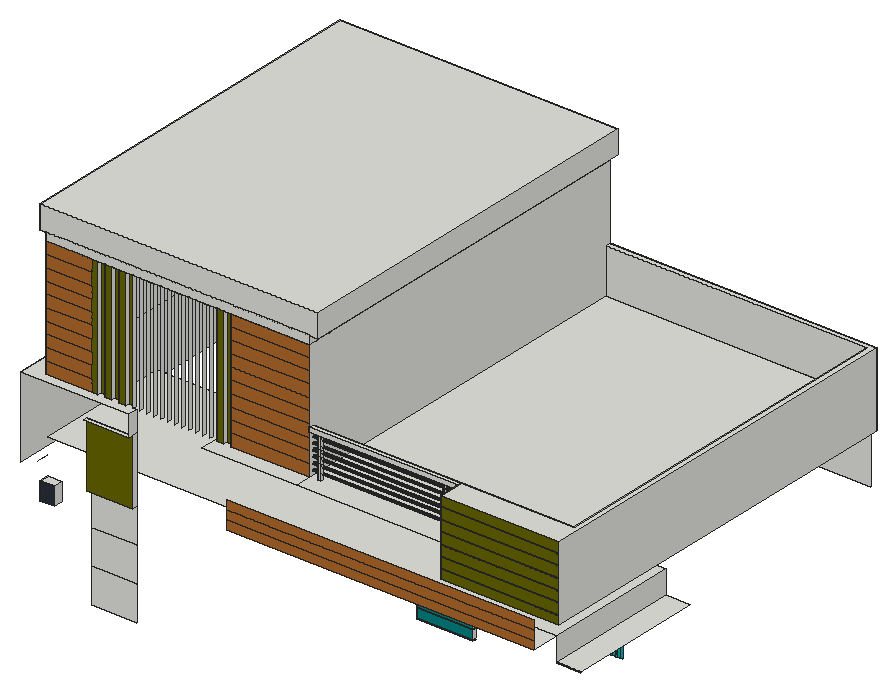
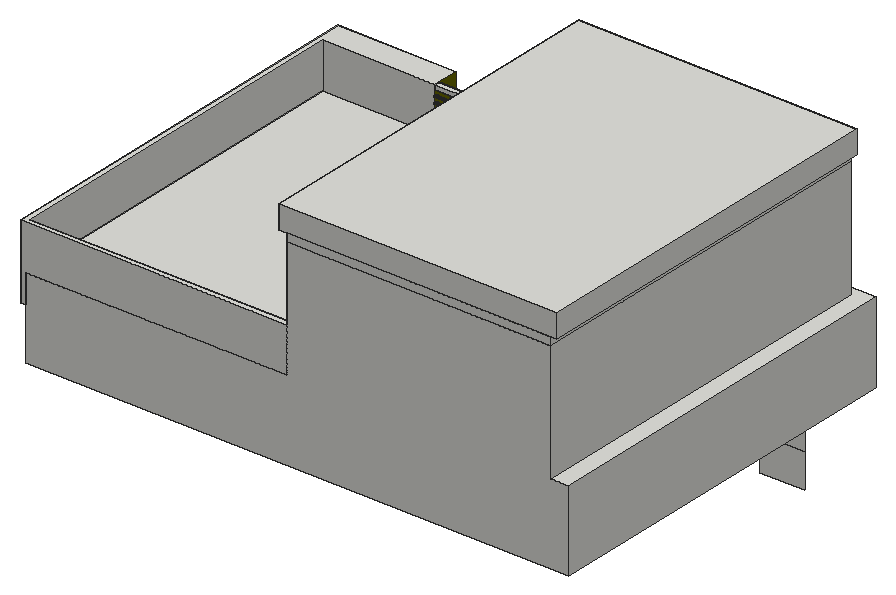
# SketchUp Ruby script. Lengths in inches.
U = 1.inch
M = Sketchup.active_model
def pt(a) = Geom::Point3d.new(a.map { |v| v * U })
def face(e, loops, mat)
  f = e.add_face(loops[0].map { |a| pt(a) })
  loops[1..].each { |l| e.add_face(l.map { |a| pt(a) }).erase! }
  f.material = f.back_material = mat if mat
  f
end
# faces: each face lists its corners as indices into pts; further lists are holes
def faces(e, pts, list, mat = nil) = list.each { |f| face(e, (f[0].is_a?(Array) ? f : [f]).map { |l| l.map { |i| pts[i] } }, mat) }
# xy, xz, yz: faces in a plane at the given z, y or x. An outline is a flat list of corners, or four numbers for a rectangle; further outlines are holes
def ring(l) = l.size == 4 ? [[l[0], l[1]], [l[2], l[1]], [l[2], l[3]], [l[0], l[3]]] : l.each_slice(2).to_a
def flat(e, list, mat, &to3) = list.each { |f| face(e, (f[0].is_a?(Array) ? f : [f]).map { |l| ring(l).map { |u, v| to3.(u, v) } }, mat) }
def xy(e, z, list, mat = nil) = flat(e, list, mat) { |x, y| [x, y, z] }
def xz(e, y, list, mat = nil) = flat(e, list, mat) { |x, z| [x, y, z] }
def yz(e, x, list, mat = nil) = flat(e, list, mat) { |y, z| [x, y, z] }
def lines(e, pts, list) = list.each { |a, b| e.add_line(pt(pts[a]), pt(pts[b])) }
# prism: a flat outline (further loops are holes) pulled along v
def prism(e, loops, v, mat = nil)
  f = face(e, loops, mat); d = Geom::Vector3d.new(v.map { |x| x * U })
  f.pushpull(f.normal.samedirection?(d) ? d.length : -d.length)
end
def box(e, o, s, mat = nil) = prism(e, [[o, [o[0] + s[0], o[1], o[2]], [o[0] + s[0], o[1] + s[1], o[2]], [o[0], o[1] + s[1], o[2]]]], [0, 0, s[2]], mat)
def at(x, y, z, deg = 0) = Geom::Transformation.translation(pt([x, y, z])) * Geom::Transformation.rotation(ORIGIN, Z_AXIS, deg.degrees)
def axes(o, x, y, z) = Geom::Transformation.new([*x, 0, *y, 0, *z, 0, *pt(o).to_a, 1])
def part(name) = M.definitions.add(name)
# library, detail: a bought-in or finely detailed component or shape, given as its bounding box
def library(name, o, s) = part(name).tap { |d| box(d.entities, o, s) }
def detail(e, o, s) = box(e.add_group.entities, o, s)
def put(e, d, t, mat = nil) = e.add_instance(d, t).tap { |i| i.material = mat if mat }
def group(e, t, mat = nil) = e.add_group.tap { |g| g.transformation = t; g.material = mat if mat }.entities
root = M.entities
M.materials.add("[Color E08]").color = [102, 102, 0]
M.materials.add("[Color H06]").color = [0, 170, 170]
M.materials.add("[Color H07]").color = [0, 132, 132]
M.materials.add("[Tile Navy]").color = [43, 47, 58]
M.materials.add("[Wood Bamboo]").color = [177, 105, 43]
xy(root,176.551,[[244.901,188.3125,281.433,190.25]])
xy(root,177.301,[[244.901,188.3125,281.433,190.25]])
xy(root,182.734,[[244.901,188.3125,281.433,190.25]])
xy(root,183.484,[[244.901,188.3125,281.433,190.25]])
xy(root,188.918,[[244.901,188.3125,281.433,190.25]])
xy(root,189.668,[[244.901,188.3125,281.433,190.25]])
xy(root,195.101,[[244.901,188.3125,281.433,190.25]])
xy(root,195.851,[[219.446,181.4375,232.76,188.3125],[244.901,188.3125,281.433,190.25]])
xy(root,201.284,[[244.901,188.3125,281.433,190.25]])
xy(root,202.034,[[244.901,188.3125,281.433,190.25]])
xy(root,207.467,[[244.901,188.3125,281.433,190.25]])
xy(root,207.989,[[308.71,183.8125,317.574,188.3125]])
xy(root,208.217,[[244.901,188.3125,281.433,190.25]])
xy(root,208.654,[[368.197,183.8125,377.586,188.3125]])
xy(root,209.164,[[219.446,181.4375,232.76,188.3125]])
xy(root,213.65,[[244.901,188.3125,281.433,190.25]])
xy(root,214.4,[[244.901,188.3125,281.433,190.25]])
xy(root,218.86,[[308.447,183.8125,323.522,188.3125],[323.522,183.8125,361.655,188.3125],[361.655,183.8125,378.322,188.3125]])
xy(root,219.833,[[244.901,188.3125,281.433,190.25]])
xy(root,220.583,[[244.901,188.3125,281.433,190.25]])
xy(root,226.016,[[244.901,188.3125,281.433,190.25]])
xy(root,226.766,[[244.901,188.3125,281.433,190.25]])
xy(root,232.199,[[244.901,188.3125,281.433,190.25]])
xy(root,232.949,[[244.901,188.3125,281.433,190.25]])
xy(root,234.298,[[308.447,183.8125,378.322,188.3125]])
xy(root,237.467,[[244.901,188.3125,281.433,190.25]])
xy(root,237.5,[[89.426,80,98.551,86.125]])
xy(root,238.982,[[243.386,188.3125,282.948,190.25]])
xy(root,239.5,[[302.454,183.8125,382.891,188.3125]])
xy(root,246.5625,[[405.1875,100.496,421.0625,188.3125]])
xy(root,247.247,[[112.439,89,141.564,92.3125]])
xy(root,249,[[89.426,80,98.551,86.125]])
xy(root,261.3125,[[207.779,82.0625,405.1875,100.496],[77.779,100.496,405.1875,188.3125]])
xy(root,284.3125,[[348.593,77.9375,348.593,82.0625,421.0625,82.0625,421.0625,333.5625,424.6875,333.5625,424.6875,77.9375]])
xy(root,289.375,[[112.439,86.125,141.564,89]])
xy(root,290,[[348.593,77.9375,424.6875,78.25]])
xy(root,290.5625,[[348.593,77.9375,424.6875,78.25]])
xy(root,297.125,[[348.593,77.9375,424.6875,78.25]])
xy(root,297.6875,[[348.593,77.9375,424.6875,78.25]])
xy(root,303,[[191.8125,82.0625,252.914,82.0625,252.914,92.3125,202.376,92.3125,202.376,94.5,197.879,94.5,197.879,92.3125,193.383,92.3125,193.383,94.5,191.8125,94.5],[[252.914,82.0625,348.593,82.0625,348.593,94.9375,421.0625,94.9375,421.0625,330.432,252.914,330.432],[257.914,93.077,259.601,94.291],[337.947,93.039,339.322,94.101]],[348.593,82.0625,421.0625,94.9375],[71.6875,86.125,141.564,86.125,141.564,92.3125,139.42,92.3125,139.42,94.5,134.923,94.5,134.923,92.3125,130.426,92.3125,130.426,94.5,125.929,94.5,125.929,92.3125,121.433,92.3125,121.433,94.5,116.936,94.5,116.936,92.3125,83.065,92.3125,83.065,333.5625,71.6875,333.5625],[252.914,330.432,421.0625,333.5625]])
xy(root,304.25,[[348.593,77.9375,424.6875,78.25]])
xy(root,304.8125,[[348.593,77.9375,424.6875,78.25]])
xy(root,311.375,[[348.593,77.9375,424.6875,78.25]])
xy(root,311.9375,[[348.593,77.9375,424.6875,78.25]])
xy(root,318.5,[[348.593,77.9375,424.6875,78.25]])
xy(root,319.0625,[[348.593,77.9375,424.6875,78.25]])
xy(root,325.625,[[348.593,77.9375,424.6875,78.25]])
xy(root,326.1875,[[348.593,77.9375,424.6875,78.25]])
xy(root,329.3125,[[[252.843,92.0625,348.593,94.9375],[257.914,93.077,259.601,94.291],[337.947,93.039,339.322,94.101]]])
xy(root,332.1875,[[348.593,77.9375,424.6875,77.9375,424.6875,333.5625,252.914,333.5625,252.914,330.432,421.0625,330.432,421.0625,94.9375,348.593,94.9375],[252.843,92.0625,348.593,94.9375]])
xy(root,379.625,[[83.065,92.3125,83.065,333.5625,252.914,333.5625,252.914,92.3125,202.376,92.3125,202.376,94.5,197.879,94.5,197.879,92.3125,193.383,92.3125,193.383,94.5,188.886,94.5,188.886,92.3125,184.389,92.3125,184.389,94.5,179.892,94.5,179.892,92.3125,175.395,92.3125,175.395,94.5,170.898,94.5,170.898,92.3125,166.401,92.3125,166.401,94.5,161.904,94.5,161.904,92.3125,157.408,92.3125,157.408,94.5,152.911,94.5,152.911,92.3125,148.414,92.3125,148.414,94.5,143.917,94.5,143.917,92.3125,139.42,92.3125,139.42,94.5,134.923,94.5,134.923,92.3125,130.426,92.3125,130.426,94.5,125.929,94.5,125.929,92.3125,121.433,92.3125,121.433,94.5,116.936,94.5,116.936,92.3125],[116.936,92.3125,121.433,94.5],[125.929,92.3125,130.426,94.5],[134.923,92.3125,139.42,94.5],[143.917,92.3125,148.414,94.5],
  [152.911,92.3125,157.408,94.5],[161.904,92.3125,166.401,94.5],[170.898,92.3125,175.395,94.5],[179.892,92.3125,184.389,94.5],[188.886,92.3125,193.383,94.5],
  [197.879,92.3125,202.376,94.5]])
xy(root,384.875,[[79.503,92.3125,83.065,333.5625],[83.065,92.3125,252.914,333.5625],[252.914,92.3125,258.539,333.5625]])
xy(root,399.875,[[79.503,92.3125,258.539,333.5625]])
xz(root,77.9375,[[348.593,284.3125,424.6875,290],[348.593,290.5625,424.6875,297.125],[348.593,297.6875,424.6875,304.25],[348.593,304.8125,424.6875,311.375],[348.593,311.9375,424.6875,318.5],
  [348.593,319.0625,424.6875,325.625],[348.593,326.1875,424.6875,332.1875]],"[Color E08]")
xz(root,78.25,[[348.593,290,424.6875,290.5625],[348.593,297.125,424.6875,297.6875],[348.593,304.25,424.6875,304.8125],[348.593,311.375,424.6875,311.9375],[348.593,318.5,424.6875,319.0625],
  [348.593,325.625,424.6875,326.1875]],"[Color E08]")
xz(root,80,[[89.426,237.5,98.551,249]],"[Tile Navy]")
xz(root,82.0625,[[348.593,284.3125,421.0625,303]])
xz(root,82.0625,[[207.779,261.3125,405.1875,266.969],[207.779,266.969,405.1875,272.828],[207.779,272.828,405.1875,278.6875]],"[Wood Bamboo]")
xz(root,89,[[112.439,247.247,141.564,289.375]],"[Color E08]")
xz(root,92.0625,[[252.843,329.3125,348.593,332.1875]])
xz(root,92.3125,[[112.439,179.96,141.564,202.389],[112.439,202.389,141.564,224.818],[112.439,224.818,141.564,247.247],[83.065,379.625,252.914,384.875],[79.503,384.875,258.539,399.875]])
xz(root,92.3125,[[112.439,303,116.936,379.625],[121.433,303,125.929,379.625],[130.426,303,134.923,379.625],[193.383,303,197.879,379.625]],"[Color E08]")
xz(root,92.3125,[[83.065,303,112.439,310.662],[202.376,303,252.914,310.662],[83.065,310.662,112.439,318.325],[202.376,310.662,252.914,318.325],[83.065,318.325,112.439,325.987],
  [202.376,318.325,252.914,325.987],[83.065,325.987,112.439,333.65],[202.376,325.987,252.914,333.65],[83.065,333.65,112.439,341.3125],[202.376,333.65,252.914,341.3125],
  [83.065,341.3125,112.439,348.975],[202.376,341.3125,252.914,348.975],[83.065,348.975,112.439,356.637],[202.376,348.975,252.914,356.637],[83.065,356.637,112.439,364.3],
  [202.376,356.637,252.914,364.3],[83.065,364.3,112.439,371.962],[202.376,364.3,252.914,371.962],[83.065,371.962,112.439,379.625],[202.376,371.962,252.914,379.625]],"[Wood Bamboo]")
xz(root,93.039,[[337.947,303,339.322,329.3125]])
xz(root,93.077,[[257.914,303,259.601,329.3125]])
xz(root,94.101,[[337.947,303,339.322,329.3125]])
xz(root,94.291,[[257.914,303,259.601,329.3125]])
xz(root,94.5,[[116.936,303,121.433,379.625],[125.929,303,130.426,379.625],[134.923,303,139.42,379.625],[197.879,303,202.376,379.625]],"[Color E08]")
xz(root,94.9375,[[348.593,303,421.0625,332.1875],[252.843,329.3125,348.593,332.1875]])
xz(root,100.496,[[405.1875,245.8125,421.0625,246.5625]])
xz(root,181.4375,[[219.446,195.851,232.76,209.164]],"[Tile Navy]")
xz(root,188.3125,[[340.843,199.631,338.019,213.116,336.94,212.694,336.4,212.484],[344.282,199.631,349.316,212.273,347.158,213.116],[308.71,199.673,309.597,207.989],[309.597,199.673,310.483,207.989],[310.483,199.673,311.369,207.989],
  [311.369,199.673,312.256,207.989],[312.256,199.673,313.142,207.989],[313.142,199.673,314.028,207.989],[314.028,199.673,314.915,207.989],[314.915,199.673,315.801,207.989],
  [315.801,199.673,316.687,207.989],[316.687,199.673,317.574,207.989],[368.197,199.914,369.24,208.654],[369.24,199.914,370.284,208.654],[370.284,199.914,371.327,208.654],
  [371.327,199.914,372.37,208.654],[372.37,199.914,373.413,208.654],[373.413,199.914,374.456,208.654],[374.456,199.914,375.5,208.654],[375.5,199.914,376.543,208.654],
  [376.543,199.914,377.586,208.654],[308.447,218.86,318.429,222.72],[318.429,218.86,328.411,222.72],[328.411,218.86,338.393,222.72],[338.393,218.86,348.376,222.72],
  [348.376,218.86,358.358,222.72],[358.358,218.86,368.34,222.72],[368.34,218.86,378.322,222.72],[308.447,222.72,318.429,226.579],[318.429,222.72,328.411,226.579],
  [328.411,222.72,338.393,226.579],[338.393,222.72,348.376,226.579],[348.376,222.72,358.358,226.579],[358.358,222.72,368.34,226.579],[368.34,222.72,378.322,226.579],
  [308.447,226.579,318.429,230.438],[318.429,226.579,328.411,230.438],[328.411,226.579,338.393,230.438],[338.393,226.579,348.376,230.438],[348.376,226.579,358.358,230.438],
  [358.358,226.579,368.34,230.438],[368.34,226.579,378.322,230.438],[308.447,230.438,318.429,234.298],[318.429,230.438,328.411,234.298],[328.411,230.438,338.393,234.298],
  [338.393,230.438,348.376,234.298],[348.376,230.438,358.358,234.298],[358.358,230.438,368.34,234.298],[368.34,230.438,378.322,234.298]],"[Color H06]")
xz(root,188.3125,[[244.901,177.301,281.433,182.734],[244.901,183.484,281.433,188.918],[244.901,189.668,281.433,195.101],[244.901,195.851,281.433,201.284],[244.901,202.034,281.433,207.467],
  [244.901,208.217,281.433,213.65],[244.901,214.4,281.433,219.833],[244.901,220.583,281.433,226.016],[244.901,226.766,281.433,232.199],[244.901,232.949,281.433,237.467]],"[Color H07]")
xz(root,330.432,[[252.914,303,421.0625,332.1875]])
xz(root,333.5625,[[71.6875,250.9375,71.6875,303,83.065,303,83.065,379.625,252.914,379.625,252.914,303,421.0625,303,421.0625,250.9375],[421.0625,284.3125,421.0625,303,252.914,303,252.914,332.1875,424.6875,332.1875,424.6875,284.3125],[83.065,379.625,252.914,384.875],[79.503,384.875,258.539,399.875]])
yz(root,71.6875,[[86.125,250.9375,333.5625,303]])
yz(root,79.503,[[92.3125,384.875,333.5625,399.875]])
yz(root,83.065,[[92.3125,303,333.5625,379.625],[92.3125,379.625,333.5625,384.875]])
yz(root,89.426,[[80,237.5,86.125,249]])
yz(root,98.551,[[80,237.5,86.125,249]])
yz(root,116.936,[[92.3125,303,94.5,379.625]])
yz(root,121.433,[[92.3125,303,94.5,379.625]])
yz(root,125.929,[[92.3125,303,94.5,379.625]])
yz(root,130.426,[[92.3125,303,94.5,379.625]])
yz(root,134.923,[[92.3125,303,94.5,379.625]])
yz(root,139.42,[[92.3125,303,94.5,379.625]])
yz(root,141.564,[[89,247.247,92.3125,289.375],[86.125,289.375,92.3125,303]])
yz(root,143.917,[[92.3125,303,94.5,379.625]])
yz(root,148.414,[[92.3125,303,94.5,379.625]])
yz(root,152.911,[[92.3125,303,94.5,379.625]])
yz(root,157.408,[[92.3125,303,94.5,379.625]])
yz(root,161.904,[[92.3125,303,94.5,379.625]])
yz(root,166.401,[[92.3125,303,94.5,379.625]])
yz(root,170.898,[[92.3125,303,94.5,379.625]])
yz(root,175.395,[[92.3125,303,94.5,379.625]])
yz(root,179.892,[[92.3125,303,94.5,379.625]])
yz(root,184.389,[[92.3125,303,94.5,379.625]])
yz(root,188.886,[[92.3125,303,94.5,379.625]])
yz(root,193.383,[[92.3125,303,94.5,379.625]])
yz(root,197.879,[[92.3125,303,94.5,379.625]])
yz(root,202.376,[[92.3125,303,94.5,379.625]])
yz(root,219.446,[[181.4375,195.851,188.3125,209.164]])
yz(root,232.76,[[181.4375,195.851,188.3125,209.164]])
yz(root,244.901,[[188.3125,177.301,190.25,182.734],[188.3125,183.484,190.25,188.918],[188.3125,189.668,190.25,195.101],[188.3125,195.851,190.25,201.284],[188.3125,202.034,190.25,207.467],
  [188.3125,208.217,190.25,213.65],[188.3125,214.4,190.25,219.833],[188.3125,220.583,190.25,226.016],[188.3125,226.766,190.25,232.199],[188.3125,232.949,190.25,237.467]])
yz(root,252.843,[[92.0625,329.3125,94.9375,332.1875]])
yz(root,252.914,[[[92.3125,303,330.432,303,330.432,332.1875,333.5625,332.1875,333.5625,379.625,92.3125,379.625],[95.1,313.411,94.939,313.432,94.788,313.494,94.658,313.594,94.559,313.723,94.497,313.874,94.475,314.036,94.497,314.197,94.559,314.348,94.658,314.478,94.788,314.577,94.939,314.639,95.1,314.661,95.262,314.639,95.413,314.577,95.542,314.478,95.642,314.348,95.704,314.197,95.725,314.036,95.704,313.874,95.642,313.723,95.542,313.594,95.413,313.494,95.262,313.432],[95.1,309.523,94.939,309.544,94.788,309.607,94.658,309.706,94.559,309.836,94.497,309.986,94.475,310.148,94.497,310.31,94.559,310.461,94.658,310.59,94.788,310.689,94.939,310.752,95.1,310.773,95.262,310.752,95.413,310.689,95.542,310.59,95.642,310.461,95.704,310.31,95.725,310.148,95.704,309.986,95.642,309.836,95.542,309.706,95.413,309.607,95.262,309.544],[95.1,325.073,94.939,325.094,94.788,325.157,94.658,325.256,94.559,325.386,94.497,325.536,94.475,325.698,94.497,325.86,94.559,326.011,94.658,326.14,94.788,326.239,94.939,326.302,95.1,326.323,95.262,326.302,95.413,326.239,95.542,326.14,95.642,326.011,95.704,325.86,95.725,325.698,95.704,325.536,95.642,325.386,95.542,325.256,95.413,325.157,95.262,325.094],[95.1,305.636,94.939,305.657,94.788,305.719,94.658,305.819,94.559,305.948,94.497,306.099,94.475,306.261,94.497,306.422,94.559,306.573,94.658,306.703,94.788,306.802,94.939,306.864,95.1,306.886,95.262,306.864,95.413,306.802,95.542,306.703,95.642,306.573,95.704,306.422,95.725,306.261,95.704,306.099,95.642,305.948,95.542,305.819,95.413,305.719,95.262,305.657],[95.1,321.186,94.939,321.207,94.788,321.269,94.658,321.369,94.559,321.498,94.497,321.649,94.475,321.811,94.497,321.972,94.559,322.123,94.658,322.253,94.788,322.352,94.939,322.414,95.1,322.436,95.262,322.414,95.413,322.352,95.542,322.253,95.642,322.123,95.704,321.972,95.725,321.811,95.704,321.649,95.642,321.498,95.542,321.369,95.413,321.269,95.262,321.207],[95.1,317.298,94.939,317.319,94.788,317.382,94.658,317.481,94.559,317.611,94.497,317.761,94.475,317.923,94.497,318.085,94.559,318.236,94.658,318.365,94.788,318.464,94.939,318.527,95.1,318.548,95.262,318.527,95.413,318.464,95.542,318.365,95.642,318.236,95.704,318.085,95.725,317.923,95.704,317.761,95.642,317.611,95.542,317.481,95.413,317.382,95.262,317.319]],[92.3125,379.625,333.5625,384.875]])
yz(root,257.914,[[93.077,303,94.291,329.3125]])
yz(root,258.539,[[92.3125,384.875,333.5625,399.875]])
yz(root,259.601,[[93.077,303,94.291,329.3125]])
yz(root,281.433,[[188.3125,177.301,190.25,182.734],[188.3125,183.484,190.25,188.918],[188.3125,189.668,190.25,195.101],[188.3125,195.851,190.25,201.284],[188.3125,202.034,190.25,207.467],
  [188.3125,208.217,190.25,213.65],[188.3125,214.4,190.25,219.833],[188.3125,220.583,190.25,226.016],[188.3125,226.766,190.25,232.199],[188.3125,232.949,190.25,237.467]])
yz(root,308.447,[[183.8125,218.86,188.3125,234.298]])
yz(root,337.947,[[93.039,303,94.101,329.3125]])
yz(root,339.322,[[93.039,303,94.101,329.3125]])
yz(root,348.593,[[95.1,305.636,95.262,305.657,95.413,305.719,95.542,305.819,95.642,305.948,95.704,306.099,95.725,306.261,95.704,306.422,95.642,306.573,95.542,306.703,95.413,306.802,95.262,306.864,95.1,306.886,94.939,306.864,94.9375,306.864,94.9375,305.657,94.939,305.657],[94.9375,305.657,94.9375,306.864,94.788,306.802,94.658,306.703,94.559,306.573,94.497,306.422,94.475,306.261,94.497,306.099,94.559,305.948,94.658,305.819,94.788,305.719],[95.1,309.523,95.262,309.544,95.413,309.607,95.542,309.706,95.642,309.836,95.704,309.986,95.725,310.148,95.704,310.31,95.642,310.461,95.542,310.59,95.413,310.689,95.262,310.752,95.1,310.773,94.939,310.752,94.9375,310.751,94.9375,309.545,94.939,309.544],[94.9375,309.545,94.9375,310.751,94.788,310.689,94.658,310.59,94.559,310.461,94.497,310.31,94.475,310.148,94.497,309.986,94.559,309.836,94.658,309.706,94.788,309.607],[95.1,313.411,95.262,313.432,95.413,313.494,95.542,313.594,95.642,313.723,95.704,313.874,95.725,314.036,95.704,314.197,95.642,314.348,95.542,314.478,95.413,314.577,95.262,314.639,95.1,314.661,94.939,314.639,94.9375,314.639,94.9375,313.432,94.939,313.432],
  [94.9375,313.432,94.9375,314.639,94.788,314.577,94.658,314.478,94.559,314.348,94.497,314.197,94.475,314.036,94.497,313.874,94.559,313.723,94.658,313.594,94.788,313.494],[95.1,317.298,95.262,317.319,95.413,317.382,95.542,317.481,95.642,317.611,95.704,317.761,95.725,317.923,95.704,318.085,95.642,318.236,95.542,318.365,95.413,318.464,95.262,318.527,95.1,318.548,94.939,318.527,94.9375,318.526,94.9375,317.32,94.939,317.319],[94.9375,317.32,94.9375,318.526,94.788,318.464,94.658,318.365,94.559,318.236,94.497,318.085,94.475,317.923,94.497,317.761,94.559,317.611,94.658,317.481,94.788,317.382],[95.1,321.186,95.262,321.207,95.413,321.269,95.542,321.369,95.642,321.498,95.704,321.649,95.725,321.811,95.704,321.972,95.642,322.123,95.542,322.253,95.413,322.352,95.262,322.414,95.1,322.436,94.939,322.414,94.9375,322.414,94.9375,321.207,94.939,321.207],[94.9375,321.207,94.9375,322.414,94.788,322.352,94.658,322.253,94.559,322.123,94.497,321.972,94.475,321.811,94.497,321.649,94.559,321.498,94.658,321.369,94.788,321.269],
  [95.1,325.073,95.262,325.094,95.413,325.157,95.542,325.256,95.642,325.386,95.704,325.536,95.725,325.698,95.704,325.86,95.642,326.011,95.542,326.14,95.413,326.239,95.262,326.302,95.1,326.323,94.939,326.302,94.9375,326.301,94.9375,325.095,94.939,325.094],[94.9375,325.095,94.9375,326.301,94.788,326.239,94.658,326.14,94.559,326.011,94.497,325.86,94.475,325.698,94.497,325.536,94.559,325.386,94.658,325.256,94.788,325.157],[92.0625,329.3125,94.9375,332.1875]])
yz(root,348.593,[[77.9375,284.3125,77.9375,290,78.25,290,78.25,290.5625,77.9375,290.5625,77.9375,297.125,78.25,297.125,78.25,297.6875,77.9375,297.6875,77.9375,304.25,78.25,304.25,78.25,304.8125,77.9375,304.8125,77.9375,311.375,78.25,311.375,78.25,311.9375,77.9375,311.9375,77.9375,318.5,78.25,318.5,78.25,319.0625,77.9375,319.0625,77.9375,325.625,78.25,325.625,78.25,326.1875,77.9375,326.1875,77.9375,332.1875,92.0625,332.1875,92.0625,329.3125,94.9375,329.3125,94.9375,326.301,94.788,326.239,94.658,326.14,94.559,326.011,94.497,325.86,94.475,325.698,94.497,325.536,94.559,325.386,94.658,325.256,94.788,325.157,94.9375,325.095,94.9375,322.414,94.788,322.352,94.658,322.253,94.559,322.123,94.497,321.972,94.475,321.811,94.497,321.649,94.559,321.498,94.658,321.369,94.788,321.269,94.9375,321.207,94.9375,318.526,94.788,318.464,94.658,318.365,94.559,318.236,94.497,318.085,94.475,317.923,94.497,317.761,94.559,317.611,94.658,317.481,94.788,317.382,94.9375,317.32,94.9375,314.639,94.788,314.577,94.658,314.478,94.559,314.348,94.497,314.197,94.475,314.036,94.497,313.874,94.559,313.723,94.658,313.594,94.788,313.494,94.9375,313.432,94.9375,310.751,94.788,310.689,94.658,310.59,94.559,310.461,94.497,310.31,94.475,310.148,94.497,309.986,94.559,309.836,94.658,309.706,94.788,309.607,94.9375,309.545,94.9375,306.864,94.788,306.802,94.658,306.703,94.559,306.573,94.497,306.422,94.475,306.261,94.497,306.099,94.559,305.948,94.658,305.819,94.788,305.719,94.9375,305.657,94.9375,303,82.0625,303,82.0625,284.3125]],"[Color E08]")
yz(root,378.322,[[183.8125,218.86,188.3125,234.298]])
yz(root,405.1875,[[100.496,246.5625,188.3125,261.3125]])
yz(root,421.0625,[[82.0625,284.3125,333.5625,303],[94.9375,303,330.432,332.1875]])
yz(root,424.6875,[[77.9375,284.3125,333.5625,284.3125,333.5625,332.1875,77.9375,332.1875,77.9375,326.1875,78.25,326.1875,78.25,325.625,77.9375,325.625,77.9375,319.0625,78.25,319.0625,78.25,318.5,77.9375,318.5,77.9375,311.9375,78.25,311.9375,78.25,311.375,77.9375,311.375,77.9375,304.8125,78.25,304.8125,78.25,304.25,77.9375,304.25,77.9375,297.6875,78.25,297.6875,78.25,297.125,77.9375,297.125,77.9375,290.5625,78.25,290.5625,78.25,290,77.9375,290]])
p = [[330.453,188.3125,207.989],[332.036,188.3125,209.681],[332.036,183.8125,209.681],[330.453,183.8125,207.989],[353.141,188.3125,209.681],[354.724,188.3125,207.989],
  [354.724,183.8125,207.989],[353.141,183.8125,209.681],[333.851,188.3125,211.12],[333.851,183.8125,211.12],[351.325,188.3125,211.12],[351.325,183.8125,211.12],
  [335.261,188.3125,211.929],[335.261,183.8125,211.929],[349.916,188.3125,211.929],[349.916,183.8125,211.929],[335.861,188.3125,212.273],[335.861,183.8125,212.273],
  [349.316,188.3125,212.273],[349.316,183.8125,212.273],[336.4,188.3125,212.484],[336.94,188.3125,212.694],[338.019,188.3125,213.116],[338.019,183.8125,213.116],
  [347.158,188.3125,213.116],[347.158,183.8125,213.116],[340.278,188.3125,213.629],[340.278,183.8125,213.629],[344.899,188.3125,213.629],[344.899,183.8125,213.629],
  [342.588,188.3125,213.801],[342.588,183.8125,213.801],[252.914,94.939,305.657],[252.914,95.1,305.636],[348.593,95.1,305.636],[348.593,94.939,305.657],
  [252.914,95.262,305.657],[348.593,95.262,305.657],[252.914,94.658,305.819],[252.914,94.788,305.719],[348.593,94.788,305.719],[348.593,94.658,305.819],
  [348.593,94.9375,305.657],[252.914,95.413,305.719],[348.593,95.413,305.719],[252.914,95.542,305.819],[348.593,95.542,305.819],[252.914,94.559,305.948],
  [348.593,94.559,305.948],[252.914,95.642,305.948],[348.593,95.642,305.948],[252.914,94.497,306.099],[348.593,94.497,306.099],[252.914,95.704,306.099],
  [348.593,95.704,306.099],[252.914,94.475,306.261],[348.593,94.475,306.261],[252.914,95.725,306.261],[348.593,95.725,306.261],[252.914,94.497,306.422],
  [348.593,94.497,306.422],[252.914,95.704,306.422],[348.593,95.704,306.422],[252.914,94.559,306.573],[348.593,94.559,306.573],[252.914,95.642,306.573],
  [348.593,95.642,306.573],[252.914,94.658,306.703],[348.593,94.658,306.703],[252.914,95.542,306.703],[348.593,95.542,306.703],[252.914,94.788,306.802],
  [348.593,94.788,306.802],[252.914,95.413,306.802],[348.593,95.413,306.802],[252.914,94.939,306.864],[348.593,94.9375,306.864],[348.593,94.939,306.864],
  [252.914,95.262,306.864],[348.593,95.262,306.864],[252.914,95.1,306.886],[348.593,95.1,306.886],[252.914,94.788,309.607],[252.914,94.939,309.544],
  [348.593,94.939,309.544],[348.593,94.9375,309.545],[348.593,94.788,309.607],[252.914,95.1,309.523],[348.593,95.1,309.523],[252.914,95.262,309.544],
  [348.593,95.262,309.544],[252.914,95.413,309.607],[348.593,95.413,309.607],[252.914,94.658,309.706],[348.593,94.658,309.706],[252.914,95.542,309.706],
  [348.593,95.542,309.706],[252.914,94.559,309.836],[348.593,94.559,309.836],[252.914,95.642,309.836],[348.593,95.642,309.836],[252.914,94.497,309.986],
  [348.593,94.497,309.986],[252.914,95.704,309.986],[348.593,95.704,309.986],[252.914,94.475,310.148],[348.593,94.475,310.148],[252.914,95.725,310.148],
  [348.593,95.725,310.148],[252.914,94.497,310.31],[348.593,94.497,310.31],[252.914,95.704,310.31],[348.593,95.704,310.31],[252.914,94.559,310.461],
  [348.593,94.559,310.461],[252.914,95.642,310.461],[348.593,95.642,310.461],[252.914,94.658,310.59],[348.593,94.658,310.59],[252.914,95.542,310.59],
  [348.593,95.542,310.59],[252.914,94.788,310.689],[348.593,94.788,310.689],[252.914,95.413,310.689],[348.593,95.413,310.689],[252.914,94.939,310.752],
  [348.593,94.9375,310.751],[348.593,94.939,310.752],[252.914,95.262,310.752],[348.593,95.262,310.752],[252.914,95.1,310.773],[348.593,95.1,310.773],
  [252.914,94.788,313.494],[252.914,94.939,313.432],[348.593,94.939,313.432],[348.593,94.9375,313.432],[348.593,94.788,313.494],[252.914,95.1,313.411],
  [348.593,95.1,313.411],[252.914,95.262,313.432],[348.593,95.262,313.432],[252.914,95.413,313.494],[348.593,95.413,313.494],[252.914,94.658,313.594],
  [348.593,94.658,313.594],[252.914,95.542,313.594],[348.593,95.542,313.594],[252.914,94.559,313.723],[348.593,94.559,313.723],[252.914,95.642,313.723],
  [348.593,95.642,313.723],[252.914,94.497,313.874],[348.593,94.497,313.874],[252.914,95.704,313.874],[348.593,95.704,313.874],[252.914,94.475,314.036],
  [348.593,94.475,314.036],[252.914,95.725,314.036],[348.593,95.725,314.036],[252.914,94.497,314.197],[348.593,94.497,314.197],[252.914,95.704,314.197],
  [348.593,95.704,314.197],[252.914,94.559,314.348],[348.593,94.559,314.348],[252.914,95.642,314.348],[348.593,95.642,314.348],[252.914,94.658,314.478],
  [348.593,94.658,314.478],[252.914,95.542,314.478],[348.593,95.542,314.478],[252.914,94.788,314.577],[348.593,94.788,314.577],[252.914,95.413,314.577],
  [348.593,95.413,314.577],[252.914,94.939,314.639],[348.593,94.9375,314.639],[348.593,94.939,314.639],[252.914,95.1,314.661],[348.593,95.1,314.661],
  [252.914,95.262,314.639],[348.593,95.262,314.639],[252.914,94.788,317.382],[252.914,94.939,317.319],[348.593,94.939,317.319],[348.593,94.9375,317.32],
  [348.593,94.788,317.382],[252.914,95.1,317.298],[348.593,95.1,317.298],[252.914,95.262,317.319],[348.593,95.262,317.319],[252.914,95.413,317.382],
  [348.593,95.413,317.382],[252.914,94.658,317.481],[348.593,94.658,317.481],[252.914,95.542,317.481],[348.593,95.542,317.481],[252.914,94.559,317.611],
  [348.593,94.559,317.611],[252.914,95.642,317.611],[348.593,95.642,317.611],[252.914,94.497,317.761],[348.593,94.497,317.761],[252.914,95.704,317.761],
  [348.593,95.704,317.761],[252.914,94.475,317.923],[348.593,94.475,317.923],[252.914,95.725,317.923],[348.593,95.725,317.923],[252.914,94.497,318.085],
  [348.593,94.497,318.085],[252.914,95.704,318.085],[348.593,95.704,318.085],[252.914,94.559,318.236],[348.593,94.559,318.236],[252.914,95.642,318.236],
  [348.593,95.642,318.236],[252.914,94.658,318.365],[348.593,94.658,318.365],[252.914,95.542,318.365],[348.593,95.542,318.365],[252.914,94.788,318.464],
  [348.593,94.788,318.464],[252.914,95.413,318.464],[348.593,95.413,318.464],[252.914,94.939,318.527],[348.593,94.9375,318.526],[348.593,94.939,318.527],
  [252.914,95.1,318.548],[348.593,95.1,318.548],[252.914,95.262,318.527],[348.593,95.262,318.527],[252.914,94.788,321.269],[252.914,94.939,321.207],
  [348.593,94.939,321.207],[348.593,94.9375,321.207],[348.593,94.788,321.269],[252.914,95.1,321.186],[348.593,95.1,321.186],[252.914,95.262,321.207],
  [348.593,95.262,321.207],[252.914,95.413,321.269],[348.593,95.413,321.269],[252.914,94.658,321.369],[348.593,94.658,321.369],[252.914,95.542,321.369],
  [348.593,95.542,321.369],[252.914,94.559,321.498],[348.593,94.559,321.498],[252.914,95.642,321.498],[348.593,95.642,321.498],[252.914,94.497,321.649],
  [348.593,94.497,321.649],[252.914,95.704,321.649],[348.593,95.704,321.649],[252.914,94.475,321.811],[348.593,94.475,321.811],[252.914,95.725,321.811],
  [348.593,95.725,321.811],[252.914,94.497,321.972],[348.593,94.497,321.972],[252.914,95.704,321.972],[348.593,95.704,321.972],[252.914,94.559,322.123],
  [348.593,94.559,322.123],[252.914,95.642,322.123],[348.593,95.642,322.123],[252.914,94.658,322.253],[348.593,94.658,322.253],[252.914,95.542,322.253],
  [348.593,95.542,322.253],[252.914,94.788,322.352],[348.593,94.788,322.352],[252.914,95.413,322.352],[348.593,95.413,322.352],[252.914,94.939,322.414],
  [348.593,94.9375,322.414],[348.593,94.939,322.414],[252.914,95.1,322.436],[348.593,95.1,322.436],[252.914,95.262,322.414],[348.593,95.262,322.414],
  [252.914,94.788,325.157],[252.914,94.939,325.094],[348.593,94.939,325.094],[348.593,94.9375,325.095],[348.593,94.788,325.157],[252.914,95.1,325.073],
  [348.593,95.1,325.073],[252.914,95.262,325.094],[348.593,95.262,325.094],[252.914,95.413,325.157],[348.593,95.413,325.157],[252.914,94.658,325.256],
  [348.593,94.658,325.256],[252.914,95.542,325.256],[348.593,95.542,325.256],[252.914,94.559,325.386],[348.593,94.559,325.386],[252.914,95.642,325.386],
  [348.593,95.642,325.386],[252.914,94.497,325.536],[348.593,94.497,325.536],[252.914,95.704,325.536],[348.593,95.704,325.536],[252.914,94.475,325.698],
  [348.593,94.475,325.698],[252.914,95.725,325.698],[348.593,95.725,325.698],[252.914,94.497,325.86],[348.593,94.497,325.86],[252.914,95.704,325.86],
  [348.593,95.704,325.86],[252.914,94.559,326.011],[348.593,94.559,326.011],[252.914,95.642,326.011],[348.593,95.642,326.011],[252.914,94.658,326.14],
  [348.593,94.658,326.14],[252.914,95.542,326.14],[348.593,95.542,326.14],[252.914,94.788,326.239],[348.593,94.788,326.239],[252.914,95.413,326.239],
  [348.593,95.413,326.239],[252.914,94.939,326.302],[348.593,94.9375,326.301],[348.593,94.939,326.302],[252.914,95.262,326.302],[348.593,95.262,326.302],
  [252.914,95.1,326.323],[348.593,95.1,326.323],[77.779,100.496,250.9375],[77.779,92.3125,250.9375]]
faces(root,p,[[0,1,2,3],[4,5,6,7],[1,8,9,2],[10,4,7,11],[8,12,13,9],[14,10,11,15],[12,16,17,13],[18,14,15,19],
  [16,20,21,22,23,17],[24,18,19,25],[22,26,27,23],[28,24,25,29],[26,30,31,27],[30,28,29,31],[32,33,34,35],[33,36,37,34],
  [38,39,40,41],[39,32,35,42,40],[36,43,44,37],[43,45,46,44],[47,38,41,48],[45,49,50,46],[51,47,48,52],[49,53,54,50],
  [55,51,52,56],[53,57,58,54],[59,55,56,60],[57,61,62,58],[63,59,60,64],[61,65,66,62],[67,63,64,68],[65,69,70,66],
  [71,67,68,72],[69,73,74,70],[75,71,72,76,77],[73,78,79,74],[80,75,77,81],[78,80,81,79],[82,83,84,85,86],[83,87,88,84],
  [87,89,90,88],[89,91,92,90],[93,82,86,94],[91,95,96,92],[97,93,94,98],[95,99,100,96],[101,97,98,102],[99,103,104,100],
  [105,101,102,106],[103,107,108,104],[109,105,106,110],[107,111,112,108],[113,109,110,114],[111,115,116,112],[117,113,114,118],[115,119,120,116],
  [121,117,118,122],[119,123,124,120],[125,121,122,126,127],[123,128,129,124],[130,125,127,131],[128,130,131,129],[132,133,134,135,136],[133,137,138,134],
  [137,139,140,138],[139,141,142,140],[143,132,136,144],[141,145,146,142],[147,143,144,148],[145,149,150,146],[151,147,148,152],[149,153,154,150],
  [155,151,152,156],[153,157,158,154],[159,155,156,160],[157,161,162,158],[163,159,160,164],[161,165,166,162],[167,163,164,168],[165,169,170,166],
  [171,167,168,172],[169,173,174,170],[175,171,172,176,177],[178,175,177,179],[180,178,179,181],[173,180,181,174],[182,183,184,185,186],[183,187,188,184],
  [187,189,190,188],[189,191,192,190],[193,182,186,194],[191,195,196,192],[197,193,194,198],[195,199,200,196],[201,197,198,202],[199,203,204,200],
  [205,201,202,206],[203,207,208,204],[209,205,206,210],[207,211,212,208],[213,209,210,214],[211,215,216,212],[217,213,214,218],[215,219,220,216],
  [221,217,218,222],[219,223,224,220],[225,221,222,226,227],[228,225,227,229],[230,228,229,231],[223,230,231,224],[232,233,234,235,236],[233,237,238,234],
  [237,239,240,238],[239,241,242,240],[243,232,236,244],[241,245,246,242],[247,243,244,248],[245,249,250,246],[251,247,248,252],[249,253,254,250],
  [255,251,252,256],[253,257,258,254],[259,255,256,260],[257,261,262,258],[263,259,260,264],[261,265,266,262],[267,263,264,268],[265,269,270,266],
  [271,267,268,272],[269,273,274,270],[275,271,272,276,277],[278,275,277,279],[280,278,279,281],[273,280,281,274],[282,283,284,285,286],[283,287,288,284],
  [287,289,290,288],[289,291,292,290],[293,282,286,294],[291,295,296,292],[297,293,294,298],[295,299,300,296],[301,297,298,302],[299,303,304,300],
  [305,301,302,306],[303,307,308,304],[309,305,306,310],[307,311,312,308],[313,309,310,314],[311,315,316,312],[317,313,314,318],[315,319,320,316],
  [321,317,318,322],[319,323,324,320],[325,321,322,326,327],[323,328,329,324],[330,325,327,331],[328,330,331,329]])
lines(root,p,[[332,333]])
